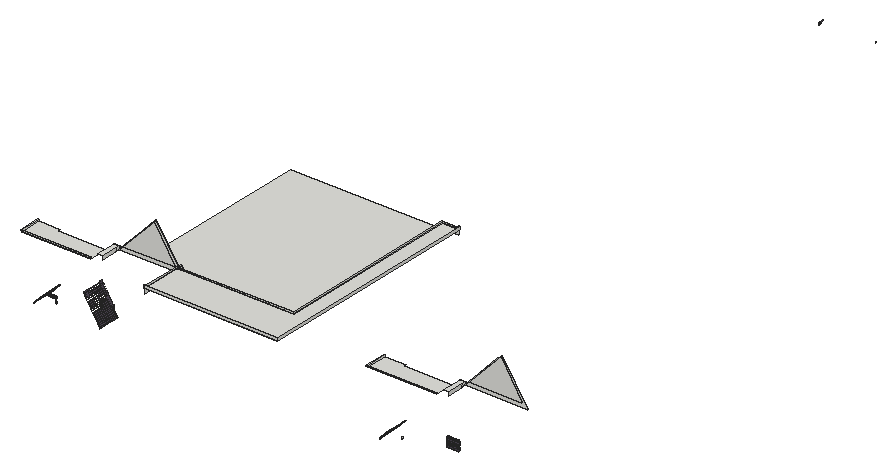
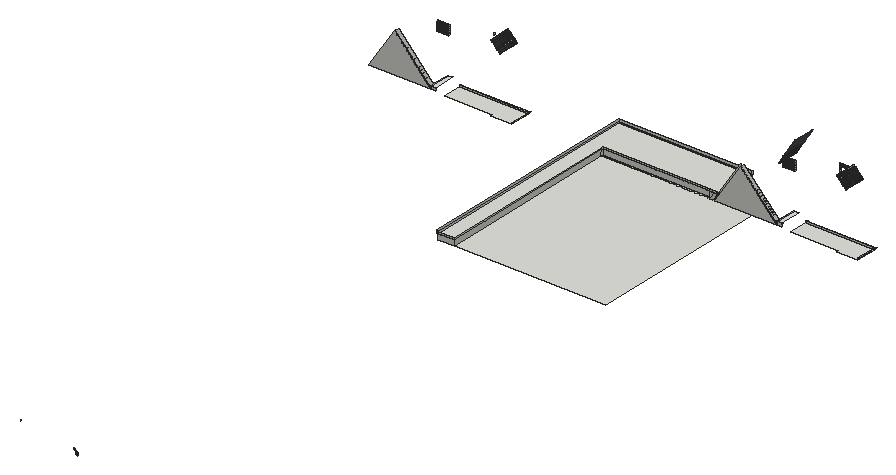
# SketchUp Ruby script. Lengths in inches.
U = 1.inch
M = Sketchup.active_model
def pt(a) = Geom::Point3d.new(a.map { |v| v * U })
def face(e, loops, mat)
  f = e.add_face(loops[0].map { |a| pt(a) })
  loops[1..].each { |l| e.add_face(l.map { |a| pt(a) }).erase! }
  f.material = f.back_material = mat if mat
  f
end
# faces: each face lists its corners as indices into pts; further lists are holes
def faces(e, pts, list, mat = nil) = list.each { |f| face(e, (f[0].is_a?(Array) ? f : [f]).map { |l| l.map { |i| pts[i] } }, mat) }
# xy, xz, yz: faces in a plane at the given z, y or x. An outline is a flat list of corners, or four numbers for a rectangle; further outlines are holes
def ring(l) = l.size == 4 ? [[l[0], l[1]], [l[2], l[1]], [l[2], l[3]], [l[0], l[3]]] : l.each_slice(2).to_a
def flat(e, list, mat, &to3) = list.each { |f| face(e, (f[0].is_a?(Array) ? f : [f]).map { |l| ring(l).map { |u, v| to3.(u, v) } }, mat) }
def xy(e, z, list, mat = nil) = flat(e, list, mat) { |x, y| [x, y, z] }
def xz(e, y, list, mat = nil) = flat(e, list, mat) { |x, z| [x, y, z] }
def yz(e, x, list, mat = nil) = flat(e, list, mat) { |y, z| [x, y, z] }
def lines(e, pts, list) = list.each { |a, b| e.add_line(pt(pts[a]), pt(pts[b])) }
# prism: a flat outline (further loops are holes) pulled along v
def prism(e, loops, v, mat = nil)
  f = face(e, loops, mat); d = Geom::Vector3d.new(v.map { |x| x * U })
  f.pushpull(f.normal.samedirection?(d) ? d.length : -d.length)
end
def box(e, o, s, mat = nil) = prism(e, [[o, [o[0] + s[0], o[1], o[2]], [o[0] + s[0], o[1] + s[1], o[2]], [o[0], o[1] + s[1], o[2]]]], [0, 0, s[2]], mat)
def at(x, y, z, deg = 0) = Geom::Transformation.translation(pt([x, y, z])) * Geom::Transformation.rotation(ORIGIN, Z_AXIS, deg.degrees)
def axes(o, x, y, z) = Geom::Transformation.new([*x, 0, *y, 0, *z, 0, *pt(o).to_a, 1])
def part(name) = M.definitions.add(name)
# library, detail: a bought-in or finely detailed component or shape, given as its bounding box
def library(name, o, s) = part(name).tap { |d| box(d.entities, o, s) }
def detail(e, o, s) = box(e.add_group.entities, o, s)
def put(e, d, t, mat = nil) = e.add_instance(d, t).tap { |i| i.material = mat if mat }
def group(e, t, mat = nil) = e.add_group.tap { |g| g.transformation = t; g.material = mat if mat }.entities
root = M.entities
M.materials.add("[Color M06]").color = [79, 71, 84]
xy(root,341.52,[[578.05,524.25,609.02,526.125],[1464.52,524.25,1495.49,526.125]])
xy(root,341.93,[[578.05,524.25,609.02,526.125],[1464.52,524.25,1495.49,526.125]])
xy(root,342.6875,[[252.64,678.64,429.58,678.64,429.58,726.125,306.21,726.125,306.21,732.2,252.64,732.2],[1139.11,678.64,1316.04,678.64,1316.04,726.125,1192.67,726.125,1192.67,732.2,1139.11,732.2]])
xy(root,345.06,[[578.05,524.25,609.02,526.125],[1464.52,524.25,1495.49,526.125]])
xy(root,346,[[578.05,524.25,609.02,526.125],[1464.52,524.25,1495.49,526.125]])
xy(root,346.3125,[[250.08,676.08,252.64,678.64],[252.64,676.08,429.58,678.64],[1136.54,676.08,1139.11,678.64],[1139.11,676.08,1316.04,678.64],[250.08,678.64,252.64,732.2],
  [1136.54,678.64,1139.11,732.2]])
xy(root,349.12,[[578.05,524.25,609.02,526.125],[1464.52,524.25,1495.49,526.125]])
xy(root,350.06,[[578.05,524.25,609.02,526.125],[1464.52,524.25,1495.49,526.125]])
xy(root,350.1875,[[637.42,726.125,910.57,732.2],[522.625,732.2,910.57,1201.875]])
xy(root,353.18,[[578.05,524.25,609.02,526.125],[1464.52,524.25,1495.49,526.125]])
xy(root,354.12,[[578.05,524.25,609.02,526.125],[1464.52,524.25,1495.49,526.125]])
xy(root,357.25,[[578.05,524.25,609.02,526.125],[1464.52,524.25,1495.49,526.125]])
xy(root,358.06,[[578.05,524.25,609.02,526.125],[1464.52,524.25,1495.49,526.125]])
xy(root,358.5,[[446.875,678.64,459.19,732.2],[1333.34,678.64,1345.65,732.2]])
xy(root,361.18,[[578.05,524.25,609.02,526.125],[1464.52,524.25,1495.49,526.125]])
xy(root,361.84,[[471.1,480.14,473.37,480.77],[473.97,480.14,476.28,480.77],[476.88,480.14,479.19,480.77],[479.79,480.14,482.1,480.77],[482.7,480.14,485.02,480.77],
  [485.61,480.14,487.93,480.77],[488.53,480.14,490.84,480.77],[491.4375,480.14,493.75,480.77],[494.35,480.14,496.66,480.77],[497.26,480.14,499.58,480.77]])
xy(root,362,[[578.05,524.25,609.02,526.125],[1464.52,524.25,1495.49,526.125]])
xy(root,363.75,[[611.36,620.41,952.01,623.84],[952.01,620.41,955.44,623.84],[611.36,623.84,611.36,726.125,910.57,726.125,910.57,1201.875,952.01,1201.875,952.01,623.84],[952.01,623.84,955.44,1201.875]])
xy(root,363.92,[[609.02,521.5625,610.9,526.125]])
xy(root,364.15,[[473.27,480.14,473.37,480.77],[473.97,480.14,476.28,480.77],[476.88,480.14,479.19,480.77],[479.79,480.14,482.1,480.77],[482.7,480.14,485.02,480.77],
  [485.61,480.14,487.93,480.77],[488.53,480.14,490.84,480.77],[491.4375,480.14,493.75,480.77],[494.35,480.14,496.66,480.77],[497.26,480.14,499.58,480.77]])
xy(root,364.65,[[473.97,480.14,476.28,480.77],[476.88,480.14,479.19,480.77],[479.79,480.14,482.1,480.77],[482.7,480.14,485.02,480.77],[485.61,480.14,487.93,480.77],
  [488.53,480.14,490.84,480.77],[491.4375,480.14,493.75,480.77],[494.35,480.14,496.66,480.77],[497.26,480.14,499.58,480.77]])
xy(root,365.12,[[578.05,524.25,608.25,526.125],[1464.52,524.25,1494.72,526.125]])
xz(root,480.77,[[497.26,350.59,499.58,352.9],[1383.73,350.59,1386.04,352.9],[497.26,353.4,499.58,355.71],[1383.73,353.4,1386.04,355.71]])
xz(root,519.6875,[[610.53,360.76,610.9,360.99,610.84,361.08,610.47,360.85],[609.84,361.83,610.21,362.07,609.02,363.92,609.02,363.11],[609.02,363.11,608.66,363.68,609.02,363.92],[608.2,364.39,608.15,364.48,608.51,364.71,608.57,364.625]])
xz(root,521.5625,[[452.05,341.69,454.48,344.27,454.02,344.7,451.6,342.125],[1338.52,341.69,1340.94,344.27,1340.48,344.7,1338.0625,342.125],[621.48,343.68,621.85,343.92,620.15,346.56,619.78,346.32],[455.35,345.2,457.77,347.77,457.32,348.2,454.9,345.63],[1341.82,345.2,1344.24,347.77,1343.78,348.2,1341.36,345.63],
  [619.15,347.3125,619.52,347.55,617.82,350.19,617.46,349.95],[458.65,348.7,461.07,351.28,460.62,351.7,458.2,349.13],[1345.12,348.7,1347.54,351.28,1347.08,351.7,1344.66,349.13],[616.82,350.94,617.19,351.18,615.5,353.82,615.13,353.58],[461.95,352.21,464.37,354.78,463.92,355.21,461.49,352.64],
  [1348.41,352.21,1350.84,354.78,1350.38,355.21,1347.96,352.64],[614.5,354.57,614.86,354.81,613.17,357.45,612.8,357.22],[465.25,355.71,467.67,358.28,467.21,358.71,464.79,356.14],[1351.71,355.71,1354.13,358.28,1353.68,358.71,1351.26,356.14],[612.17,358.2,612.54,358.4375,610.9,360.99,610.9,360.18],
  [468.55,359.22,470.97,361.79,470.51,362.22,468.09,359.64],[1355.01,359.22,1357.43,361.79,1356.98,362.22,1354.56,359.64],[610.9,360.18,610.53,360.76,610.9,360.99],[610.9,360.99,610.9,363.92,609.02,363.92,610.21,362.07,610.84,361.08],[471.85,362.72,474.27,365.29,473.8125,365.72,471.39,363.15],
  [1358.31,362.72,1360.73,365.29,1360.28,365.72,1357.85,363.15],[608.66,363.68,608.2,364.39,608.57,364.625,609.02,363.92],[607.51,365.46,605.875,368.02,606.24,368.25,607.88,365.7]])
xz(root,524.25,[[578.05,341.93,609.02,345.06],[1464.52,341.93,1495.49,345.06],[578.05,346,609.02,349.12],[1464.52,346,1495.49,349.12],[578.05,350.06,609.02,353.18],
  [1464.52,350.06,1495.49,353.18],[578.05,354.12,609.02,357.25],[1464.52,354.12,1495.49,357.25],[578.05,358.06,609.02,361.18],[1464.52,358.06,1495.49,361.18],
  [578.05,362,609.02,362,609.02,363.92,608.25,365.12,578.05,365.12]],"[Color M06]")
xz(root,526.125,[[578.05,341.52,609.02,341.93],[1464.52,341.52,1495.49,341.93],[578.05,345.06,609.02,346],[1464.52,345.06,1495.49,346],[578.05,349.12,609.02,350.06],
  [1464.52,349.12,1495.49,350.06],[578.05,353.18,609.02,354.12],[1464.52,353.18,1495.49,354.12],[578.05,357.25,609.02,358.06],[1464.52,357.25,1495.49,358.06],
  [578.05,361.18,609.02,362],[1464.52,361.18,1495.49,362],[609.02,363.92,609.02,365.12,608.25,365.12],[578.05,365.12,608.25,365.12,607.53,366.25,578.05,366.25],[1464.52,365.12,1494.72,365.12,1494,366.25,1464.52,366.25]])
xz(root,620.41,[[611.36,363.75,955.44,370.8125]])
xz(root,623.84,[[611.36,363.75,952.01,367.1875]])
xz(root,678.64,[[252.64,342.6875,429.58,346.3125],[1139.11,342.6875,1316.04,346.3125]])
xz(root,726.125,[[611.36,350.1875,611.36,360.28,617.83,350.1875],[617.83,350.1875,617.83,359.1,614.85,363.75,611.36,363.75,611.36,360.28],[617.83,350.1875,623.54,350.1875,617.83,359.1],[623.54,350.1875,617.83,359.1,617.83,363.75,623.54,363.75],[623.54,350.1875,637.42,363.75],
  [637.42,350.1875,910.57,363.75],[617.83,359.1,614.85,363.75,617.83,363.75],[611.36,360.28,611.36,364.9375,608.37,364.9375],[611.36,363.75,611.36,364.9375,614.09,364.9375,614.85,363.75],[614.85,363.75,614.09,364.9375,612.64,367.1875,614.85,367.1875],
  [614.85,363.75,617.83,367.1875],[617.83,363.75,623.54,367.1875],[623.54,363.75,637.42,367.1875],[637.42,363.75,910.57,367.1875],[473.07,364.9375,553.56,450.4375,608.37,364.9375],
  [608.37,364.9375,553.56,450.4375,557.61,453.03,612.42,367.53,611.88,367.1875,611.36,367.1875,611.36,366.85],[608.37,364.9375,611.36,366.85,611.36,364.9375],[611.36,364.9375,611.36,366.85,611.88,367.1875,612.64,367.1875,614.09,364.9375],[1359.54,364.9375,1440.02,450.4375,1494.83,364.9375]])
xz(root,731.75,[[446.875,357.04,446.15,357.73,446.875,358.5],[1333.34,357.04,1332.61,357.73,1333.34,358.5]])
xz(root,732.2,[[630.97,340.75,635.26,343.5,630.97,350.1875],[623.54,341.27,623.54,350.1875,617.83,350.1875],[446.875,350.1875,459.19,358.5],[459.19,350.1875,553.56,450.4375,617.83,350.1875],[623.54,350.1875,614.09,364.9375,619.35,368.3125,630.97,350.1875],
  [1333.34,350.1875,1345.65,358.5],[1345.65,350.1875,1440.02,450.4375,1504.29,350.1875],[614.09,364.9375,612.42,367.53,617.68,370.91,619.35,368.3125]])
xz(root,1201.875,[[910.57,350.1875,952.01,363.75],[910.57,363.75,952.01,367.1875],[952.01,363.75,955.44,370.8125]])
xz(root,2319.18,[[1128.57,361.83,1128.94,362.07,1127.25,364.71,1126.88,364.48]],"[Color M06]")
xz(root,2332.13,[[972.3125,343.14,973.55,344.46,972.3125,344.46],[972.3125,344.96,974.02,344.96,974.625,345.61,974.625,347.27,973.55,347.27,972.3125,345.96],[974.02,344.96,974.625,344.96,974.625,345.61],[975.23,346.25,976.1875,347.27,975.23,347.27],[975.23,347.77,976.65,347.77,977.54,348.72,977.54,350.09,976.1875,350.09,975.23,349.0625],
  [976.65,347.77,977.54,347.77,977.54,348.72]])
xz(root,2332.13,[[972.3125,345.96,973.55,347.27,972.3125,347.27],[972.3125,347.77,972.32,347.77,974.5,350.09,973.55,350.09,972.3125,348.77],[972.3125,347.77,974.02,347.77,974.625,348.42,974.625,350.09,974.5,350.09,975.23,350.86,975.23,350.59,976.65,350.59,977.54,351.53,977.54,352.9,977.15,352.9,978.14,353.95,978.14,353.4,979.29,353.4,980.45,354.64,980.45,355.71,979.79,355.71,980.26,356.21,979.29,356.21,980.45,357.45,980.45,356.41,980.26,356.21,979.79,355.71,978.82,355.71,978.14,354.98,978.14,353.95,977.15,352.9,976.1875,352.9,975.23,351.875,975.23,350.86,974.5,350.09,973.55,350.09,972.3125,348.77],[972.32,347.77,974.02,347.77,974.625,348.42,974.625,350.09,974.5,350.09],[974.02,347.77,974.625,347.77,974.625,348.42]],"[Color M06]")
yz(root,252.64,[[678.64,342.6875,732.2,346.3125]])
yz(root,459.19,[[678.64,350.1875,719.59,358.5],[719.59,350.1875,731.75,358.5],[731.75,350.1875,732.2,358.5]])
yz(root,473.37,[[480.14,361.84,480.77,364.15]])
yz(root,473.97,[[480.14,361.84,480.77,364.15],[480.14,364.65,480.77,364.89]])
yz(root,476.28,[[480.14,361.84,480.77,364.15],[480.14,364.65,480.77,366.96]])
yz(root,476.88,[[480.14,361.84,480.77,364.15],[480.14,364.65,480.77,366.96]])
yz(root,479.19,[[480.14,361.84,480.77,364.15],[480.14,364.65,480.77,366.96]])
yz(root,479.79,[[480.14,361.84,480.77,364.15],[480.14,364.65,480.77,366.96]])
yz(root,482.1,[[480.14,361.84,480.77,364.15],[480.14,364.65,480.77,366.96]])
yz(root,482.7,[[480.14,361.84,480.77,364.15],[480.14,364.65,480.77,366.96]])
yz(root,485.02,[[480.14,361.84,480.77,364.15],[480.14,364.65,480.77,366.96]])
yz(root,485.61,[[480.14,361.84,480.77,364.15],[480.14,364.65,480.77,366.96]])
yz(root,487.93,[[480.14,361.84,480.77,364.15],[480.14,364.65,480.77,366.96]])
yz(root,488.53,[[480.14,361.84,480.77,364.15],[480.14,364.65,480.77,366.96]])
yz(root,490.84,[[480.14,361.84,480.77,364.15],[480.14,364.65,480.77,366.96]])
yz(root,491.4375,[[480.14,361.84,480.77,364.15],[480.14,364.65,480.77,366.96]])
yz(root,493.75,[[480.14,361.84,480.77,364.15],[480.14,364.65,480.77,366.96]])
yz(root,494.35,[[480.14,361.84,480.77,364.15],[480.14,364.65,480.77,366.96]])
yz(root,496.66,[[480.14,361.84,480.77,364.15],[480.14,364.65,480.77,366.96]])
yz(root,497.26,[[480.14,361.84,480.77,364.15],[480.14,364.65,480.77,366.96]])
yz(root,499.58,[[480.14,361.84,480.77,364.15],[480.14,364.65,480.77,366.96]])
yz(root,578.05,[[524.25,341.93,526.125,345.06],[524.25,346,526.125,349.12],[524.25,350.06,526.125,353.18],[524.25,354.12,526.125,357.25],[524.25,358.06,526.125,361.18],
  [524.25,362,526.125,365.12]])
yz(root,609.02,[[524.25,341.93,526.125,345.06],[524.25,346,526.125,349.12],[524.25,350.06,526.125,353.18],[524.25,354.12,526.125,357.25],[524.25,358.06,526.125,361.18],
  [524.25,362,526.125,363.92]])
yz(root,611.36,[[623.84,350.1875,726.125,363.75],[620.41,363.75,623.84,370.8125],[623.84,363.75,726.125,367.1875]])
yz(root,910.57,[[726.125,350.1875,732.2,363.75],[732.2,350.1875,1201.875,363.75],[726.125,363.75,732.2,367.1875],[732.2,363.75,1201.875,367.1875]])
yz(root,952.01,[[623.84,363.75,1201.875,367.1875]])
yz(root,955.44,[[620.41,363.75,1201.875,370.8125]])
yz(root,1139.11,[[678.64,342.6875,732.2,346.3125]])
yz(root,1345.65,[[678.64,350.1875,719.59,358.5],[719.59,350.1875,731.75,358.5],[731.75,350.1875,732.2,358.5]])
yz(root,1464.52,[[524.25,341.93,526.125,345.06],[524.25,346,526.125,349.12],[524.25,350.06,526.125,353.18],[524.25,354.12,526.125,357.25],[524.25,358.06,526.125,361.18],
  [524.25,362,526.125,365.12]])
p = [[450.72,521.5625,341.19],[450.72,467.1875,341.19],[451.18,467.1875,340.76],[451.18,521.5625,340.76],[1337.1875,521.5625,341.19],[1337.1875,467.1875,341.19],
  [1337.64,467.1875,340.76],[1337.64,521.5625,340.76],[451.6,521.5625,342.125],[451.6,467.1875,342.125],[1338.0625,521.5625,342.125],[1338.0625,467.1875,342.125],
  [452.05,521.5625,341.69],[452.05,467.1875,341.69],[454.48,521.5625,344.27],[454.48,467.1875,344.27],[1338.52,521.5625,341.69],[1338.52,467.1875,341.69],
  [1340.94,521.5625,344.27],[1340.94,467.1875,344.27],[622.48,467.1875,342.93],[622.48,521.5625,342.93],[622.11,521.5625,342.69],[622.11,467.1875,342.69],
  [621.85,467.1875,343.92],[621.85,521.5625,343.92],[619.78,521.5625,346.32],[621.48,521.5625,343.68],[621.48,467.1875,343.68],[619.78,467.1875,346.32],
  [454.02,521.5625,344.7],[454.02,467.1875,344.7],[1340.48,521.5625,344.7],[1340.48,467.1875,344.7],[454.9,521.5625,345.63],[454.9,467.1875,345.63],
  [1341.36,521.5625,345.63],[1341.36,467.1875,345.63],[455.35,521.5625,345.2],[455.35,467.1875,345.2],[457.77,521.5625,347.77],[457.77,467.1875,347.77],
  [1341.82,521.5625,345.2],[1341.82,467.1875,345.2],[1344.24,521.5625,347.77],[1344.24,467.1875,347.77],[620.15,467.1875,346.56],[620.15,521.5625,346.56],
  [619.52,467.1875,347.55],[619.52,521.5625,347.55],[617.46,521.5625,349.95],[619.15,521.5625,347.3125],[619.15,467.1875,347.3125],[617.46,467.1875,349.95],
  [457.32,521.5625,348.2],[457.32,467.1875,348.2],[1343.78,521.5625,348.2],[1343.78,467.1875,348.2],[458.2,521.5625,349.13],[458.2,467.1875,349.13],
  [1344.66,521.5625,349.13],[1344.66,467.1875,349.13],[458.65,521.5625,348.7],[458.65,467.1875,348.7],[461.07,521.5625,351.28],[461.07,467.1875,351.28],
  [1345.12,521.5625,348.7],[1345.12,467.1875,348.7],[1347.54,521.5625,351.28],[1347.54,467.1875,351.28],[617.82,467.1875,350.19],[617.82,521.5625,350.19],
  [617.19,467.1875,351.18],[617.19,521.5625,351.18],[553.56,731.75,450.4375],[459.19,731.75,350.1875],[459.19,719.59,350.1875],[553.56,719.59,450.4375],
  [553.56,726.125,450.4375],[1440.02,731.75,450.4375],[1345.65,731.75,350.1875],[1345.65,719.59,350.1875],[1440.02,719.59,450.4375],[1440.02,726.125,450.4375],
  [553.56,732.2,450.4375],[459.19,732.2,350.1875],[1440.02,732.2,450.4375],[1345.65,732.2,350.1875],[615.13,521.5625,353.58],[616.82,521.5625,350.94],
  [616.82,467.1875,350.94],[615.13,467.1875,353.58],[460.62,521.5625,351.7],[460.62,467.1875,351.7],[1347.08,521.5625,351.7],[1347.08,467.1875,351.7],
  [461.49,521.5625,352.64],[461.49,467.1875,352.64],[1347.96,521.5625,352.64],[1347.96,467.1875,352.64],[461.95,521.5625,352.21],[461.95,467.1875,352.21],
  [464.37,521.5625,354.78],[464.37,467.1875,354.78],[1348.41,521.5625,352.21],[1348.41,467.1875,352.21],[1350.84,521.5625,354.78],[1350.84,467.1875,354.78],
  [615.5,467.1875,353.82],[615.5,521.5625,353.82],[614.86,467.1875,354.81],[614.86,521.5625,354.81],[612.8,521.5625,357.22],[614.5,521.5625,354.57],
  [614.5,467.1875,354.57],[612.8,467.1875,357.22],[463.92,521.5625,355.21],[463.92,467.1875,355.21],[1350.38,521.5625,355.21],[1350.38,467.1875,355.21],
  [464.79,521.5625,356.14],[464.79,467.1875,356.14],[1351.26,521.5625,356.14],[1351.26,467.1875,356.14],[465.25,521.5625,355.71],[465.25,480.14,355.71],
  [465.25,467.1875,355.71],[467.67,521.5625,358.28],[467.67,467.1875,358.28],[1351.71,521.5625,355.71],[1351.71,480.14,355.71],[1351.71,467.1875,355.71],
  [1354.13,521.5625,358.28],[1354.13,467.1875,358.28],[613.17,467.1875,357.45],[613.17,521.5625,357.45],[612.54,467.1875,358.4375],[612.54,521.5625,358.4375],
  [610.47,467.1875,360.85],[610.47,519.6875,360.85],[610.53,519.6875,360.76],[610.53,521.5625,360.76],[610.9,521.5625,360.18],[612.17,521.5625,358.2],
  [612.17,467.1875,358.2],[467.21,521.5625,358.71],[467.21,467.1875,358.71],[1353.68,521.5625,358.71],[1353.68,467.1875,358.71],[468.09,521.5625,359.64],
  [468.09,467.1875,359.64],[1354.56,521.5625,359.64],[1354.56,467.1875,359.64],[468.55,521.5625,359.22],[468.55,467.1875,359.22],[470.97,521.5625,361.79],
  [470.97,467.1875,361.79],[1355.01,521.5625,359.22],[1355.01,467.1875,359.22],[1357.43,521.5625,361.79],[1357.43,467.1875,361.79],[610.84,467.1875,361.08],
  [610.84,519.6875,361.08],[610.9,519.6875,360.99],[610.9,521.5625,360.99],[610.84,521.5625,361.08],[610.21,467.1875,362.07],[610.21,519.6875,362.07],
  [610.21,521.5625,362.07],[470.51,521.5625,362.22],[470.51,467.1875,362.22],[608.15,467.1875,364.48],[608.15,519.6875,364.48],[608.2,519.6875,364.39],
  [608.2,521.5625,364.39],[608.66,521.5625,363.68],[608.66,519.6875,363.68],[609.02,519.6875,363.11],[609.84,519.6875,361.83],[609.84,467.1875,361.83],
  [1356.98,521.5625,362.22],[1356.98,467.1875,362.22],[473.27,480.14,364.15],[471.1,480.14,361.84],[471.1,480.77,361.84],[473.27,480.77,364.15],
  [608.51,467.1875,364.71],[608.51,519.6875,364.71],[608.51,521.5625,364.71],[608.57,521.5625,364.625],[609.02,521.5625,363.92],[609.02,519.6875,363.92],
  [471.39,521.5625,363.15],[471.39,467.1875,363.15],[1357.85,521.5625,363.15],[1357.85,467.1875,363.15],[471.85,521.5625,362.72],[471.85,467.1875,362.72],
  [474.27,521.5625,365.29],[474.27,467.1875,365.29],[1358.31,521.5625,362.72],[1358.31,467.1875,362.72],[1360.73,521.5625,365.29],[1360.73,467.1875,365.29],
  [609.02,524.25,363.92],[607.88,467.1875,365.7],[607.88,521.5625,365.7],[606.24,521.5625,368.25],[606.24,519.6875,368.25],[606.1875,519.6875,368.34],
  [606.1875,467.1875,368.34],[605.55,467.1875,369.33],[605.55,521.5625,369.33],[603.92,521.5625,371.88],[603.92,519.6875,371.88],[603.86,519.6875,371.97],
  [603.86,467.1875,371.97],[603.36,467.1875,372.75],[603.36,521.5625,372.75],[601.72,521.5625,375.3],[601.72,519.6875,375.3],[601.67,519.6875,375.39],
  [601.67,467.1875,375.39],[601.17,467.1875,376.17],[601.17,521.5625,376.17],[599.53,521.5625,378.72],[599.53,519.6875,378.72],[599.47,519.6875,378.8125],
  [599.47,467.1875,378.8125],[598.98,467.1875,379.59],[598.98,521.5625,379.59],[597.34,521.5625,382.14],[597.34,519.6875,382.14],[597.28,519.6875,382.23],
  [597.28,467.1875,382.23],[596.78,467.1875,383.01],[596.78,521.5625,383.01],[595.15,521.5625,385.56],[595.15,519.6875,385.56],[595.09,519.6875,385.65],
  [595.09,467.1875,385.65],[594.59,467.1875,386.43],[594.59,521.5625,386.43],[592.95,521.5625,388.98],[592.95,519.6875,388.98],[592.9,519.6875,389.07],
  [592.9,467.1875,389.07],[592.4,467.1875,389.85],[592.4,521.5625,389.85],[590.76,521.5625,392.4],[590.76,519.6875,392.4],[590.7,519.6875,392.49],
  [590.7,467.1875,392.49],[590.21,467.1875,393.27],[590.21,521.5625,393.27],[588.57,521.5625,395.82],[588.57,519.6875,395.82],[588.51,519.6875,395.91],
  [588.51,467.1875,395.91],[588.01,467.1875,396.69],[588.01,521.5625,396.69],[586.375,521.5625,399.24],[586.375,519.6875,399.24],[586.32,519.6875,399.33],
  [586.32,467.1875,399.33],[585.82,467.1875,400.11],[585.82,521.5625,400.11],[584.18,521.5625,402.66],[584.18,519.6875,402.66],[584.125,519.6875,402.75],
  [584.125,467.1875,402.75],[583.63,467.1875,403.53],[583.63,521.5625,403.53],[581.99,521.5625,406.08],[581.99,519.6875,406.08],[581.93,519.6875,406.17],
  [581.93,467.1875,406.17],[581.44,467.1875,406.95],[581.44,521.5625,406.95],[579.8,521.5625,409.5],[579.8,519.6875,409.5],[579.74,519.6875,409.59],
  [579.74,467.1875,409.59],[579.24,467.1875,410.37],[579.24,521.5625,410.37],[578.05,521.5625,412.22],[578.05,526.125,412.22],[578.12,526.125,412.12],
  [580.125,526.125,409],[581,526.125,407.62],[581,524.25,407.62],[583.01,524.25,404.5],[583.01,526.125,404.5],[583.73,526.125,403.37],
  [583.73,524.25,403.37],[585.73,524.25,400.25],[585.73,526.125,400.25],[586.45,526.125,399.12],[586.45,524.25,399.12],[588.46,524.25,396],
  [588.46,526.125,396],[589.18,526.125,394.87],[589.18,524.25,394.87],[591.18,524.25,391.75],[591.18,526.125,391.75],[591.9,526.125,390.62],
  [591.9,524.25,390.62],[593.91,524.25,387.5],[593.91,526.125,387.5],[594.63,526.125,386.37],[594.63,524.25,386.37],[596.63,524.25,383.25],
  [596.63,526.125,383.25],[597.35,526.125,382.12],[597.35,524.25,382.12],[599.36,524.25,379],[599.36,526.125,379],[600.08,526.125,377.87],
  [600.08,524.25,377.87],[602.08,524.25,374.75],[602.08,526.125,374.75],[602.8,526.125,373.62],[602.8,524.25,373.62],[604.81,524.25,370.5],
  [604.81,526.125,370.5],[605.53,526.125,369.37],[605.53,524.25,369.37],[607.53,524.25,366.25],[607.53,526.125,366.25],[608.25,526.125,365.12],
  [608.25,524.25,365.12],[609.02,526.125,363.92],[608.57,519.6875,364.625],[475.91,480.14,366.96],[473.97,480.14,364.89],[473.97,480.77,364.89],
  [475.91,480.77,366.96],[612.64,726.125,367.1875],[612.42,726.125,367.53],[612.42,732.2,367.53],[614.09,732.2,364.9375],[614.09,726.125,364.9375],
  [473.8125,521.5625,365.72],[473.8125,467.1875,365.72],[1360.28,521.5625,365.72],[1360.28,467.1875,365.72],[605.82,467.1875,368.11],[605.82,519.6875,368.11],
  [605.875,519.6875,368.02],[605.875,521.5625,368.02],[607.51,521.5625,365.46],[607.51,467.1875,365.46],[474.6875,521.5625,366.65],[474.6875,467.1875,366.65],
  [1361.15,521.5625,366.65],[1361.15,467.1875,366.65],[1353.62,726.125,364.9375],[1436.82,726.125,453.34],[1333.34,731.75,358.5],[1334.07,731.75,357.81],
  [446.875,731.75,358.5],[447.61,731.75,357.81],[467.15,726.125,364.9375],[550.36,726.125,453.34],[977.54,2332.13,356.21],[976.65,2332.13,356.21],
  [972.32,2332.13,350.59],[972.3125,2332.13,350.59],[986.27,2332.13,365.41],[986.27,2332.13,365.35],[983.96,2332.13,362.9],[983.96,2332.13,364.15],
  [985.09,2332.13,364.15],[985.14,2332.13,364.15],[980.32,2332.13,361.84],[980.26,2332.13,361.84],[982.97,2332.13,361.84],[982.91,2332.13,361.84],
  [985.61,2332.13,364.65],[985.56,2332.13,364.65],[980.45,2332.13,359.22],[980.45,2332.13,359.17],[980.32,2332.13,359.02],[980.26,2332.13,359.02],
  [983.96,2332.13,360.14],[983.96,2332.13,361.2]]
faces(root,p,[[0,1,2,3],[4,5,6,7],[20,21,22,23],[25,24,28,27],[35,34,38,39],[37,36,42,43],[46,47,26,29],[49,48,52,51],
  [59,58,62,63],[61,60,66,67],[70,71,50,53],[74,75,76,77,78],[79,80,81,82,83],[84,85,75,74],[86,87,80,79],[73,72,90,89],
  [97,96,100,101],[99,98,104,105],[108,109,88,91],[111,110,114,113],[121,120,124,125,126],[123,122,129,130,131],[134,135,112,115],[137,136,144,143],
  [150,149,153,154],[152,151,157,158],[161,162,139,138],[163,164,141,140],[163,162,165,164],[162,167,168,165],[167,166,179,178],[182,183,184,185],
  [166,186,187,188,189,190,191,167],[190,168,167,191],[193,192,196,197],[195,194,200,201],[190,191,176,175],[329,331,204,330],[332,189,174,173],[186,187,172,171],
  [333,334,335,336],[337,338,339,340,341],[342,343,199,198],[344,345,203,202],[206,205,351,350]])
faces(root,p,[[0,8,9,1],[4,10,11,5],[9,8,12,13],[12,14,15,13],[11,10,16,17],[16,18,19,17],[20,24,25,21],[26,27,28,29],
  [30,31,15,14],[32,33,19,18],[30,34,35,31],[32,36,37,33],[38,40,41,39],[42,44,45,43],[46,48,49,47],[50,51,52,53],
  [54,55,41,40],[56,57,45,44],[54,58,59,55],[56,60,61,57],[62,64,65,63],[66,68,69,67],[70,72,73,71],[88,89,90,91],
  [92,93,65,64],[94,95,69,68],[92,96,97,93],[94,98,99,95],[100,102,103,101],[104,106,107,105],[108,110,111,109],[112,113,114,115],
  [116,117,103,102],[118,119,107,106],[116,120,121,117],[118,122,123,119],[124,127,128,126,125],[129,132,133,131,130],[134,136,137,135],[138,139,140,141,142,143,144],
  [145,146,128,127],[147,148,133,132],[145,149,150,146],[147,151,152,148],[153,155,156,154],[157,159,160,158],[161,166,167,162],[169,170,156,155],
  [171,172,173,174,175,176,177,178,179],[180,181,160,159],[169,192,193,170],[180,194,195,181],[196,198,199,197],[200,202,203,201],[204,190,189,188,187,186,205,206,207,208,209,210,211,212,213,214,215,216,217,218,219,220,221,222,223,224,225,226,227,228,229,230,231,232,233,234,235,236,237,238,239,240,241,242,243,244,245,246,247,248,249,250,251,252,253,254,255,256,257,258,259,260,261,262,263,264,265,266,267,268,269,270,271,272,273,274,275,276,277,278,279,280,281,282,283,284,285,286,287,288,289,290,291,292,293,294,295,296,297,298,299,300,301,302,303,304,305,306,307,308,309,310,311,312,313,314,315,316,317,318,319,320,321,322,323,324,325,326,327,328,329,330],[346,347,348,349,350,351],
  [342,352,353,343],[344,354,355,345]],"[Color M06]")
lines(root,p,[[356,357],[358,359],[360,361],[362,363],[364,365],[366,367],[368,369],[370,371],[372,373],[374,375],[376,377],[378,379],
  [380,381],[382,383],[384,385]])
